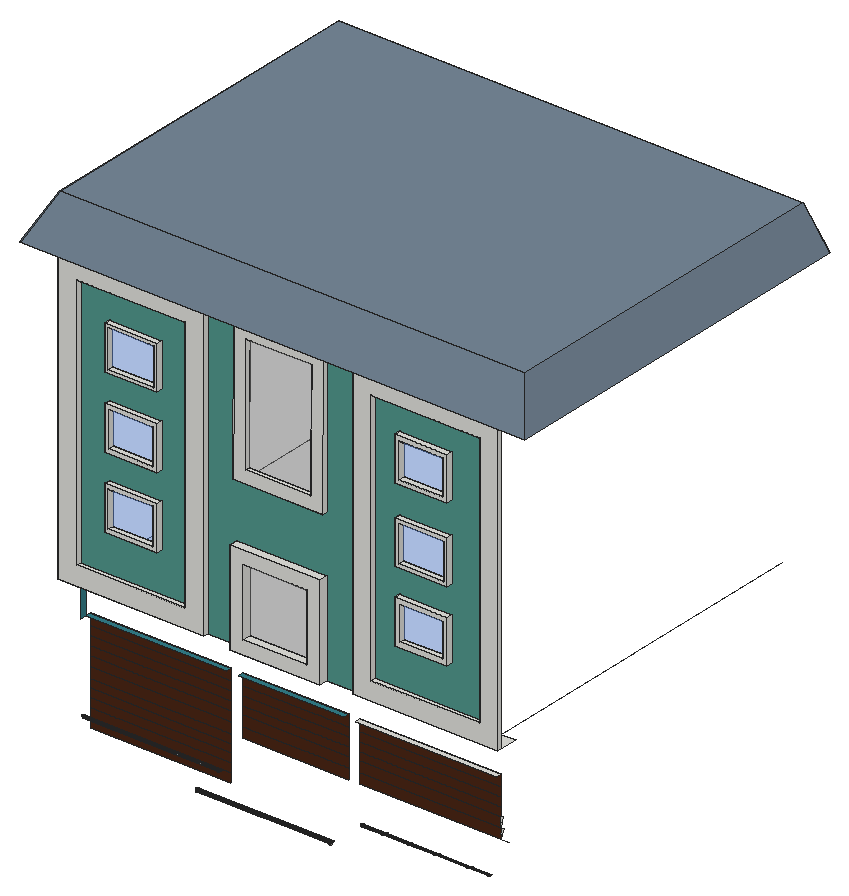
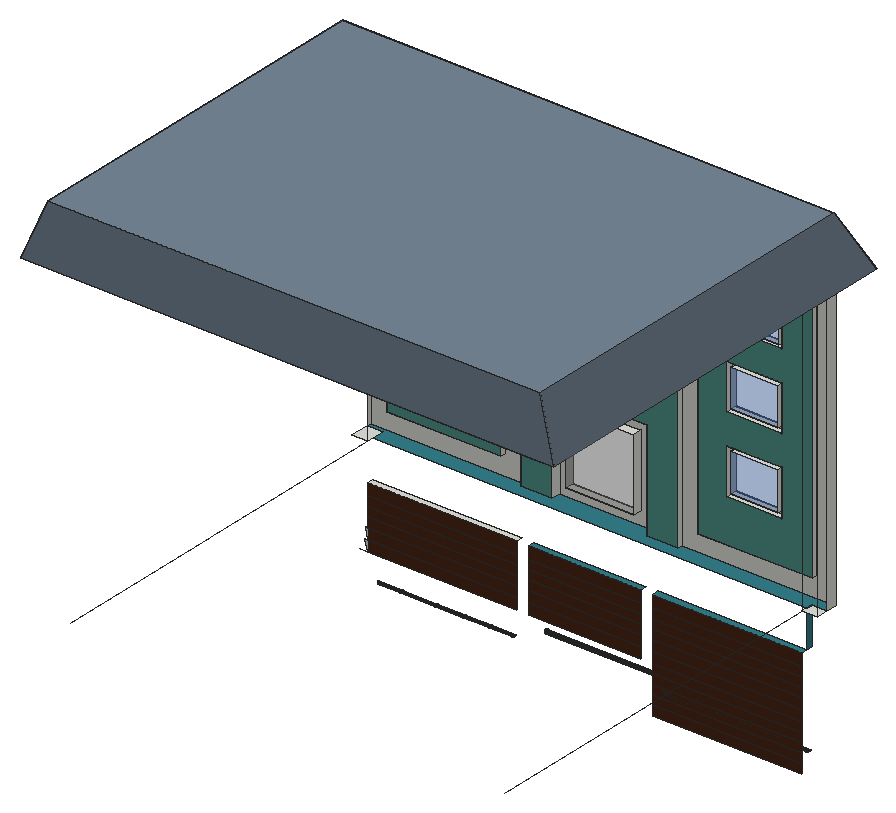
# SketchUp Ruby script. Lengths in inches.
U = 1.inch
M = Sketchup.active_model
def pt(a) = Geom::Point3d.new(a.map { |v| v * U })
def face(e, loops, mat)
  f = e.add_face(loops[0].map { |a| pt(a) })
  loops[1..].each { |l| e.add_face(l.map { |a| pt(a) }).erase! }
  f.material = f.back_material = mat if mat
  f
end
# faces: each face lists its corners as indices into pts; further lists are holes
def faces(e, pts, list, mat = nil) = list.each { |f| face(e, (f[0].is_a?(Array) ? f : [f]).map { |l| l.map { |i| pts[i] } }, mat) }
# xy, xz, yz: faces in a plane at the given z, y or x. An outline is a flat list of corners, or four numbers for a rectangle; further outlines are holes
def ring(l) = l.size == 4 ? [[l[0], l[1]], [l[2], l[1]], [l[2], l[3]], [l[0], l[3]]] : l.each_slice(2).to_a
def flat(e, list, mat, &to3) = list.each { |f| face(e, (f[0].is_a?(Array) ? f : [f]).map { |l| ring(l).map { |u, v| to3.(u, v) } }, mat) }
def xy(e, z, list, mat = nil) = flat(e, list, mat) { |x, y| [x, y, z] }
def xz(e, y, list, mat = nil) = flat(e, list, mat) { |x, z| [x, y, z] }
def yz(e, x, list, mat = nil) = flat(e, list, mat) { |y, z| [x, y, z] }
def lines(e, pts, list) = list.each { |a, b| e.add_line(pt(pts[a]), pt(pts[b])) }
# prism: a flat outline (further loops are holes) pulled along v
def prism(e, loops, v, mat = nil)
  f = face(e, loops, mat); d = Geom::Vector3d.new(v.map { |x| x * U })
  f.pushpull(f.normal.samedirection?(d) ? d.length : -d.length)
end
def box(e, o, s, mat = nil) = prism(e, [[o, [o[0] + s[0], o[1], o[2]], [o[0] + s[0], o[1] + s[1], o[2]], [o[0], o[1] + s[1], o[2]]]], [0, 0, s[2]], mat)
def at(x, y, z, deg = 0) = Geom::Transformation.translation(pt([x, y, z])) * Geom::Transformation.rotation(ORIGIN, Z_AXIS, deg.degrees)
def axes(o, x, y, z) = Geom::Transformation.new([*x, 0, *y, 0, *z, 0, *pt(o).to_a, 1])
def part(name) = M.definitions.add(name)
# library, detail: a bought-in or finely detailed component or shape, given as its bounding box
def library(name, o, s) = part(name).tap { |d| box(d.entities, o, s) }
def detail(e, o, s) = box(e.add_group.entities, o, s)
def put(e, d, t, mat = nil) = e.add_instance(d, t).tap { |i| i.material = mat if mat }
def group(e, t, mat = nil) = e.add_group.tap { |g| g.transformation = t; g.material = mat if mat }.entities
root = M.entities
M.materials.add("[0042_Sienna]").color = [76, 39, 21]
M.materials.add("[0083_DarkTurquoise]").color = [52, 127, 137]
M.materials.add("[0087_Cyan]").color = [82, 153, 141]
M.materials.add("[0110_LightSlateGray]").color = [119, 136, 153]
M.materials.add("[Steel Brushed Stainless]").color = [183, 187, 190]
M.materials.add("[Stone Marble]").color = [143, 138, 136]
M.materials.add("[Translucent Glass Blue]").color = [100, 149, 237]
M.materials["[Translucent Glass Blue]"].alpha = 0.5
M.materials.add("[Translucent Glass Gray]").color = [128, 128, 128]
M.materials["[Translucent Glass Gray]"].alpha = 0.5
xy(root,213.19,[[400.07,41.47,400.58,41.54,401.07,41.74,401.48,42.05,401.8,42.47,402,42.95,402.07,43.47,402,43.99,401.8,44.47,401.48,44.88,401.07,45.2,400.58,45.4,400.07,45.47,399.55,45.4,399.07,45.2,398.65,44.88,398.33,44.47,398.13,43.99,398.07,43.47,398.13,42.95,398.33,42.47,398.65,42.05,399.07,41.74,399.55,41.54]],"[Stone Marble]")
xy(root,213.56,[[674.75,40.78,675.26,40.84,675.75,41.04,676.16,41.36,676.48,41.78,676.68,42.26,676.75,42.78,676.68,43.29,676.48,43.78,676.16,44.19,675.75,44.51,675.26,44.71,674.75,44.78,674.23,44.71,673.75,44.51,673.33,44.19,673.01,43.78,672.8125,43.29,672.75,42.78,672.8125,42.26,673.01,41.78,673.33,41.36,673.75,41.04,674.23,40.84]],"[Stone Marble]")
xy(root,408,[[672,109.2,960,121.2]])
xy(root,408,[[120,109.2,408,121.2],[432,109.2,648,121.2]],"[0083_DarkTurquoise]")
xy(root,480,[[960,83.89,990,121.2],[90,97.2,120,121.2]])
xy(root,480,[[447.88,67.2,447.88,85.2,387.88,85.2,387.88,76.2,90,76.2,90,97.2,120,97.2,120,109.2,960,109.2,960,83.89,990,83.89,990,76.2,692.12,76.2,692.12,85.2,632.12,85.2,632.12,67.2]],"[0083_DarkTurquoise]")
xy(root,506.53,[[474.41,67.2,605.59,85.2]])
xy(root,518.4,[[128.4,76.2,349.48,85.2],[730.52,76.2,951.6,85.2]])
xy(root,601.25,[[187.24,73.2,294.0625,85.2],[781.18,73.2,888,85.2]])
xy(root,608.64,[[194.63,73.2,286.68,85.2]])
xy(root,610.87,[[790.8,73.2,878.38,85.2]])
xy(root,645.47,[[474.41,67.2,605.59,85.2]])
xy(root,672,[[447.88,67.2,632.12,85.2]])
xy(root,680.79,[[790.8,73.2,878.38,85.2]])
xy(root,683.02,[[194.63,73.2,286.68,85.2]])
xy(root,690.41,[[187.24,73.2,294.0625,85.2],[781.18,73.2,888,85.2]])
xy(root,746.69,[[781.18,73.2,888,85.2]])
xy(root,747.88,[[187.24,73.2,294.0625,85.2]])
xy(root,754.07,[[788.56,73.2,880.62,85.2]])
xy(root,755.87,[[195.24,73.2,286.07,85.2]])
xy(root,788.2,[[447.88,76.2,632.12,85.2]])
xy(root,813.27,[[473.03,76.2,607.13,85.2]])
xy(root,828.47,[[788.56,73.2,880.62,85.2]])
xy(root,829.04,[[195.24,73.2,286.07,85.2]])
xy(root,835.85,[[781.18,73.2,888,85.2]])
xy(root,837.03,[[187.24,73.2,294.0625,85.2]])
xy(root,894.88,[[187.24,73.2,294.0625,85.2]])
xy(root,900.25,[[781.18,73.2,888,85.2]])
xy(root,900.64,[[193,73.2,288.31,85.2]])
xy(root,909.0625,[[789.99,73.2,879.19,85.2]])
xy(root,978.28,[[193,73.2,288.31,85.2]])
xy(root,980.6,[[789.99,73.2,879.19,85.2]])
xy(root,984.03,[[187.24,73.2,294.0625,85.2]])
xy(root,989.41,[[781.18,73.2,888,85.2]])
xy(root,1041.6,[[128.4,76.2,349.48,85.2],[730.52,76.2,951.6,85.2]])
xy(root,1054.93,[[473.81,76.2,607.9,85.2]])
xy(root,1080,[[24,61.2,24,841.2,60,841.2,60,97.2,90,97.2,90,76.2,387.88,76.2,387.88,85.2,448.82,85.2,448.82,76.2,633.05,76.2,633.05,85.2,692.12,85.2,692.12,76.2,990,76.2,990,83.89,1020,83.89,1020,841.2,1056,841.2,1056,61.2],[90,76.2,90,97.2,60,97.2,60,841.2,1020,841.2,1020,83.89,990,83.89,990,76.2,692.12,76.2,692.12,85.2,633.05,85.2,633.05,76.2,448.82,76.2,448.82,85.2,387.88,85.2,387.88,76.2]])
xy(root,1176,[[75.68,98.82,1026.87,810.625]],"[0110_LightSlateGray]")
xz(root,67.2,[[[447.88,480,632.12,672],[474.41,506.53,605.59,645.47]]])
xz(root,73.2,[[[187.24,601.25,294.0625,690.41],[194.63,608.64,286.68,683.02]],[[781.18,601.25,888,690.41],[790.8,610.87,878.38,680.79]],[[781.18,746.69,888,835.85],[788.56,754.07,880.62,828.47]],[[187.24,747.88,294.0625,837.03],[195.24,755.87,286.07,829.04]],[[187.24,894.88,294.0625,984.03],[193,900.64,288.31,978.28]],
  [[781.18,900.25,888,989.41],[789.99,909.0625,879.19,980.6]]])
xz(root,76.2,[[[90,480,387.88,1080],[128.4,518.4,349.48,1041.6]],[[692.12,480,990,1080],[730.52,518.4,951.6,1041.6]],[[447.88,788.2,632.12,788.2,633.05,1080,448.82,1080],[473.03,813.27,473.81,1054.93,607.9,1054.93,607.13,813.27]]])
xz(root,85.2,[[387.88,480,447.88,480,447.88,672,632.12,672,632.12,480,692.12,480,692.12,1080,633.05,1080,632.12,788.2,447.88,788.2,448.82,1080,387.88,1080],[[128.4,518.4,349.48,1041.6],[187.24,601.25,294.0625,690.41],[187.24,747.88,294.0625,837.03],[187.24,894.88,294.0625,984.03]],[[730.52,518.4,951.6,1041.6],[781.18,900.25,888,989.41],[781.18,746.69,888,835.85],[781.18,601.25,888,690.41]]],"[0087_Cyan]")
xz(root,85.2,[[194.63,608.64,286.68,683.02],[790.8,610.87,878.38,680.79],[788.56,754.07,880.62,828.47],[195.24,755.87,286.07,829.04],[193,900.64,288.31,978.28],
  [789.99,909.0625,879.19,980.6]],"[Translucent Glass Blue]")
xz(root,85.2,[[474.41,506.53,605.59,645.47],[473.03,813.27,607.13,813.27,607.9,1054.93,473.81,1054.93]],"[Translucent Glass Gray]")
xz(root,121.2,[[960,288,965.375,309.1875,960,309.1875],[960,309.1875,964.0625,330,960,330]])
xz(root,121.2,[[120,198,408,216],[120,216,408,234],[120,234,408,252],[120,252,408,270],[120,270,408,288],
  [120,288,408,309.1875],[432,288,648,309.1875],[672,288,960,309.1875],[120,309.1875,408,330],[432,309.1875,648,330],
  [672,309.1875,960,330],[120,330,408,348],[432,330,648,330,648,348.12,432,348],[672,330,960,348],[120,348,408,366],
  [432,348,648,348.12,648,366,432,366],[672,348,960,366],[120,366,408,384],[432,366,648,384],[672,366,960,384],
  [120,384,408,408],[432,384,648,408],[672,384,960,408]],"[0042_Sienna]")
yz(root,90,[[76.2,480,97.2,1080]])
yz(root,120,[[97.2,408,109.2,480]],"[0083_DarkTurquoise]")
yz(root,128.4,[[76.2,518.4,85.2,1041.6]])
yz(root,187.24,[[73.2,601.25,85.2,690.41],[73.2,747.88,85.2,837.03],[73.2,894.88,85.2,984.03]])
yz(root,193,[[73.2,900.64,85.2,978.28]])
yz(root,194.63,[[73.2,608.64,85.2,683.02]])
yz(root,195.24,[[73.2,755.87,85.2,829.04]])
yz(root,286.07,[[73.2,755.87,85.2,829.04]])
yz(root,286.68,[[73.2,608.64,85.2,683.02]])
yz(root,288.31,[[73.2,900.64,85.2,978.28]])
yz(root,294.0625,[[73.2,601.25,85.2,690.41],[73.2,747.88,85.2,837.03],[73.2,894.88,85.2,984.03]])
yz(root,349.48,[[76.2,518.4,85.2,1041.6]])
yz(root,387.88,[[76.2,480,85.2,1080]])
yz(root,447.88,[[67.2,480,85.2,672]])
yz(root,474.41,[[67.2,506.53,85.2,645.47]])
yz(root,605.59,[[67.2,506.53,85.2,645.47]])
yz(root,632.12,[[67.2,480,85.2,672]])
yz(root,692.12,[[76.2,480,85.2,1080]])
yz(root,730.52,[[76.2,518.4,85.2,1041.6]])
yz(root,781.18,[[73.2,601.25,85.2,690.41],[73.2,746.69,85.2,835.85],[73.2,900.25,85.2,989.41]])
yz(root,788.56,[[73.2,754.07,85.2,828.47]])
yz(root,789.99,[[73.2,909.0625,85.2,980.6]])
yz(root,790.8,[[73.2,610.87,85.2,680.79]])
yz(root,878.38,[[73.2,610.87,85.2,680.79]])
yz(root,879.19,[[73.2,909.0625,85.2,980.6]])
yz(root,880.62,[[73.2,754.07,85.2,828.47]])
yz(root,888,[[73.2,601.25,85.2,690.41],[73.2,746.69,85.2,835.85],[73.2,900.25,85.2,989.41]])
yz(root,951.6,[[76.2,518.4,85.2,1041.6]])
yz(root,990,[[76.2,480,83.89,1080]])
p = [[400.07,43.47,213.19],[400.14,44.23,213.01],[674.51,44.23,213.01],[674.58,43.47,213.19],[402.07,43.47,213.19],[400.125,45.01,213.04],
  [674.53,45.01,213.04],[400.01,45.76,213.27],[674.64,45.76,213.27],[399.9,42.78,213.56],[674.75,42.78,213.56],[672.75,42.78,213.56],
  [631.68,42.78,213.56],[627.68,42.78,213.56],[575.31,42.78,213.56],[571.31,42.78,213.56],[525.25,42.78,213.56],[521.25,42.78,213.56],
  [464.31,42.78,213.56],[460.31,42.78,213.56],[399.81,46.43,213.68],[674.83,46.43,213.68],[399.65,42.2,214.09],[674.98,42.2,214.09],
  [399.54,46.96,214.26],[675.1,46.96,214.26],[399.34,41.79,214.76],[675.28,41.79,214.76],[399.22,47.33,214.95],[675.42,47.33,214.95],
  [398.99,41.5625,215.51],[675.62,41.5625,215.51],[398.86,47.51,215.71],[675.76,47.51,215.71],[398.63,41.54,216.29],[675.97,41.54,216.29],
  [398.49,47.48,216.49],[676.12,47.48,216.49],[398.27,41.71,217.05],[676.32,41.71,217.05],[398.14,47.25,217.24],[676.46,47.25,217.24],
  [397.94,42.08,217.74],[676.64,42.08,217.74],[397.84,46.84,217.91],[676.76,46.84,217.91],[397.67,42.62,218.32],[676.9,42.62,218.32],
  [397.59,46.27,218.44],[676.99,46.27,218.44],[397.47,43.28,218.73],[677.1,43.28,218.73],[397.42,45.57,218.81],[677.15,45.57,218.81],
  [397.36,44.03,218.96],[677.21,44.03,218.96],[397.34,44.8125,218.99],[677.23,44.8125,218.99],[402.47,100.37,226],[402.54,99.85,226.07],
  [123.86,99.85,226.07],[123.93,100.37,226],[402.54,100.88,226.07],[123.86,100.88,226.07],[692.4,102.16,226],[735.53,102.16,226],
  [735.59,101.64,226.0625],[692.34,101.64,226.0625],[786.97,101.64,226.0625],[786.9,102.16,226],[841.72,101.64,226.0625],[841.65,102.16,226],
  [909.22,101.64,226.0625],[909.15,102.16,226],[952.09,101.64,226.0625],[952.03,102.16,226],[692.33,102.67,226.07],[735.6,102.67,226.07],
  [786.98,102.67,226.07],[841.73,102.67,226.07],[909.23,102.67,226.07],[952.1,102.67,226.07],[402.74,99.37,226.27],[123.66,99.37,226.27],
  [402.74,101.37,226.27],[123.66,101.37,226.27],[735.79,101.15,226.26],[692.15,101.15,226.26],[787.16,101.15,226.26],[841.91,101.15,226.26],
  [909.41,101.15,226.26],[952.29,101.15,226.26],[692.125,103.15,226.28],[735.81,103.15,226.28],[787.18,103.15,226.28],[841.93,103.15,226.28],
  [909.43,103.15,226.28],[952.31,103.15,226.28],[403.06,98.95,226.59],[123.35,98.95,226.59],[736.1,100.74,226.57],[691.83,100.74,226.57],
  [787.47,100.74,226.57],[842.22,100.74,226.57],[909.72,100.74,226.57],[952.6,100.74,226.57],[403.06,101.78,226.59],[123.35,101.78,226.59],
  [691.8,103.56,226.6],[736.13,103.56,226.6],[787.51,103.56,226.6],[842.26,103.56,226.6],[909.76,103.56,226.6],[952.63,103.56,226.6],
  [403.47,98.63,227],[122.93,98.63,227],[736.51,100.41,226.98],[691.42,100.41,226.98],[787.88,100.41,226.98],[842.63,100.41,226.98],
  [910.13,100.41,226.98],[953.01,100.41,226.98],[403.47,102.1,227],[122.93,102.1,227],[691.38,103.88,227.02],[736.55,103.88,227.02],
  [787.92,103.88,227.02],[842.67,103.88,227.02],[910.17,103.88,227.02],[953.05,103.88,227.02],[403.95,98.43,227.48],[122.45,98.43,227.48],
  [736.99,100.21,227.46],[690.94,100.21,227.46],[788.36,100.21,227.46],[843.11,100.21,227.46],[910.61,100.21,227.46],[953.49,100.21,227.46],
  [403.95,102.3,227.48],[122.45,102.3,227.48],[690.9,104.07,227.5],[737.03,104.07,227.5],[788.41,104.07,227.5],[843.16,104.07,227.5],
  [910.66,104.07,227.5],[953.53,104.07,227.5],[404.47,98.37,228],[121.93,98.37,228],[737.51,100.13,227.98],[690.43,100.13,227.98],
  [788.88,100.13,227.98],[843.63,100.13,227.98],[911.13,100.13,227.98],[954.01,100.13,227.98],[404.47,102.37,228],[121.93,102.37,228],
  [690.38,104.13,228.02],[737.55,104.13,228.02],[788.93,104.13,228.02],[843.68,104.13,228.02],[911.18,104.13,228.02],[954.05,104.13,228.02],
  [404.99,98.43,228.52],[121.41,98.43,228.52],[738.02,100.2,228.5],[689.91,100.2,228.5],[789.4,100.2,228.5],[844.15,100.2,228.5],
  [911.65,100.2,228.5],[954.52,100.2,228.5],[404.99,102.3,228.52],[121.41,102.3,228.52],[689.86,104.0625,228.54],[738.07,104.0625,228.54],
  [789.44,104.0625,228.54],[844.19,104.0625,228.54],[911.69,104.0625,228.54],[954.57,104.0625,228.54],[405.47,98.63,229],[120.93,98.63,229],
  [738.51,100.39,228.98],[689.42,100.39,228.98],[789.88,100.39,228.98],[844.63,100.39,228.98],[912.13,100.39,228.98],[955.01,100.39,228.98],
  [405.47,102.1,229],[120.93,102.1,229],[689.38,103.86,229.02],[738.55,103.86,229.02],[789.92,103.86,229.02],[844.67,103.86,229.02],
  [912.17,103.86,229.02],[955.05,103.86,229.02],[405.89,98.95,229.41],[120.52,98.95,229.41],[738.93,100.7,229.4],[689.01,100.7,229.4],
  [790.3,100.7,229.4],[845.05,100.7,229.4],[912.55,100.7,229.4],[955.43,100.7,229.4],[405.89,101.78,229.41],[120.52,101.78,229.41],
  [688.97,103.53,229.43],[738.96,103.53,229.43],[790.33,103.53,229.43],[845.08,103.53,229.43],[912.58,103.53,229.43],[955.46,103.53,229.43],
  [406.2,99.37,229.73],[120.2,99.37,229.73],[739.25,101.12,229.72],[688.68,101.12,229.72],[790.625,101.12,229.72],[845.375,101.12,229.72],
  [912.875,101.12,229.72],[955.75,101.12,229.72],[406.2,101.37,229.73],[120.2,101.37,229.73],[688.66,103.12,229.74],[739.27,103.12,229.74],
  [790.65,103.12,229.74],[845.4,103.12,229.74],[912.9,103.12,229.74],[955.77,103.12,229.74],[406.4,99.85,229.93],[120,99.85,229.93],
  [406.4,100.88,229.93],[120,100.88,229.93],[739.45,101.6,229.93],[688.48,101.6,229.93],[790.83,101.6,229.93],[845.58,101.6,229.93],
  [913.08,101.6,229.93],[955.95,101.6,229.93],[688.47,102.63,229.9375],[739.47,102.63,229.9375],[790.84,102.63,229.9375],[845.59,102.63,229.9375],
  [913.09,102.63,229.9375],[955.97,102.63,229.9375],[406.47,100.37,230],[119.93,100.37,230],[739.53,102.11,230],[688.4,102.11,230],
  [790.9,102.11,230],[845.65,102.11,230],[913.15,102.11,230],[956.03,102.11,230],[448.82,85.2,1080],[447.88,85.2,788.2],
  [447.88,76.2,788.2],[448.82,76.2,1080],[632.12,85.2,788.2],[633.05,85.2,1080],[633.05,76.2,1080],[632.12,76.2,788.2],
  [473.03,85.2,813.27],[473.81,85.2,1054.93],[473.81,76.2,1054.93],[473.03,76.2,813.27],[607.9,85.2,1054.93],[607.13,85.2,813.27],
  [607.13,76.2,813.27],[607.9,76.2,1054.93],[1056,61.2,1080],[1026.87,98.82,1176],[75.68,98.82,1176],[24,61.2,1080],
  [75.68,810.625,1176],[24,841.2,1080],[1056,841.2,1080],[1026.87,810.625,1176],[1020,841.2,1080],[60,841.2,1080],
  [120,841.2,480],[120,121.2,480],[960,121.2,480],[960,841.2,480],[120,121.2,1080],[960,121.2,1080],
  [90,121.2,480],[90,121.2,1080],[690.4,102.13,228],[954.03,102.13,228],[121.93,100.37,228],[404.47,100.37,228],
  [398.74,44.52,216],[675.87,44.52,216],[960,121.2,288],[976.125,121.2,288]]
faces(root,p,[[0,1,2,3,4],[1,5,6,2],[5,7,8,6],[9,0,4,3,10,11,12,13,14,15,16,17,18,19],[7,20,21,8],[22,9,19,18,17,16,15,14,13,12,11,10,23],[20,24,25,21],[26,22,23,27],
  [24,28,29,25],[30,26,27,31],[28,32,33,29],[34,30,31,35],[32,36,37,33],[38,34,35,39],[36,40,41,37],[42,38,39,43],
  [40,44,45,41],[46,42,43,47],[44,48,49,45],[50,46,47,51],[48,52,53,49],[54,50,51,55],[52,56,57,53],[56,54,55,57],
  [58,59,60,61],[62,58,61,63],[64,65,66,67],[68,66,65,69],[70,68,69,71],[72,70,71,73],[74,72,73,75],[76,77,65,64],
  [69,65,77,78],[71,69,78,79],[73,71,79,80],[75,73,80,81],[59,82,83,60],[84,62,63,85],[67,66,86,87],[88,86,66,68],
  [89,88,68,70],[90,89,70,72],[91,90,72,74],[92,93,77,76],[78,77,93,94],[79,78,94,95],[80,79,95,96],[81,80,96,97],
  [82,98,99,83],[87,86,100,101],[102,100,86,88],[103,102,88,89],[104,103,89,90],[105,104,90,91],[106,84,85,107],[108,109,93,92],
  [94,93,109,110],[95,94,110,111],[96,95,111,112],[97,96,112,113],[98,114,115,99],[101,100,116,117],[118,116,100,102],[119,118,102,103],
  [120,119,103,104],[121,120,104,105],[122,106,107,123],[124,125,109,108],[110,109,125,126],[111,110,126,127],[112,111,127,128],[113,112,128,129],
  [114,130,131,115],[117,116,132,133],[134,132,116,118],[135,134,118,119],[136,135,119,120],[137,136,120,121],[138,122,123,139],[140,141,125,124],
  [126,125,141,142],[127,126,142,143],[128,127,143,144],[129,128,144,145],[130,146,147,131],[133,132,148,149],[150,148,132,134],[151,150,134,135],
  [152,151,135,136],[153,152,136,137],[154,138,139,155],[156,157,141,140],[142,141,157,158],[143,142,158,159],[144,143,159,160],[145,144,160,161],
  [146,162,163,147],[149,148,164,165],[166,164,148,150],[167,166,150,151],[168,167,151,152],[169,168,152,153],[170,154,155,171],[172,173,157,156],
  [158,157,173,174],[159,158,174,175],[160,159,175,176],[161,160,176,177],[162,178,179,163],[165,164,180,181],[182,180,164,166],[183,182,166,167],
  [184,183,167,168],[185,184,168,169],[186,170,171,187],[188,189,173,172],[174,173,189,190],[175,174,190,191],[176,175,191,192],[177,176,192,193],
  [178,194,195,179],[181,180,196,197],[198,196,180,182],[199,198,182,183],[200,199,183,184],[201,200,184,185],[202,186,187,203],[204,205,189,188],
  [190,189,205,206],[191,190,206,207],[192,191,207,208],[193,192,208,209],[194,210,211,195],[197,196,212,213],[214,212,196,198],[215,214,198,199],
  [216,215,199,200],[217,216,200,201],[218,202,203,219],[220,221,205,204],[206,205,221,222],[207,206,222,223],[208,207,223,224],[209,208,224,225],
  [210,226,227,211],[228,218,219,229],[213,212,230,231],[232,230,212,214],[233,232,214,215],[234,233,215,216],[235,234,216,217],[236,237,221,220],
  [222,221,237,238],[223,222,238,239],[224,223,239,240],[225,224,240,241],[226,242,243,227],[242,228,229,243],[231,230,244,245],[246,244,230,232],
  [247,246,232,233],[248,247,233,234],[249,248,234,235],[245,244,237,236],[238,237,244,246],[239,238,246,247],[240,239,247,248],[241,240,248,249]],"[Steel Brushed Stainless]")
faces(root,p,[[250,251,252,253],[254,255,256,257],[258,259,260,261],[262,263,264,265]])
faces(root,p,[[266,267,268,269],[269,268,270,271],[266,272,273,267],[274,275,271,270,273,272]],"[0110_LightSlateGray]")
lines(root,p,[[276,277],[278,279],[277,280],[278,281],[282,283],[284,285],[286,287],[288,289],[290,291]])
